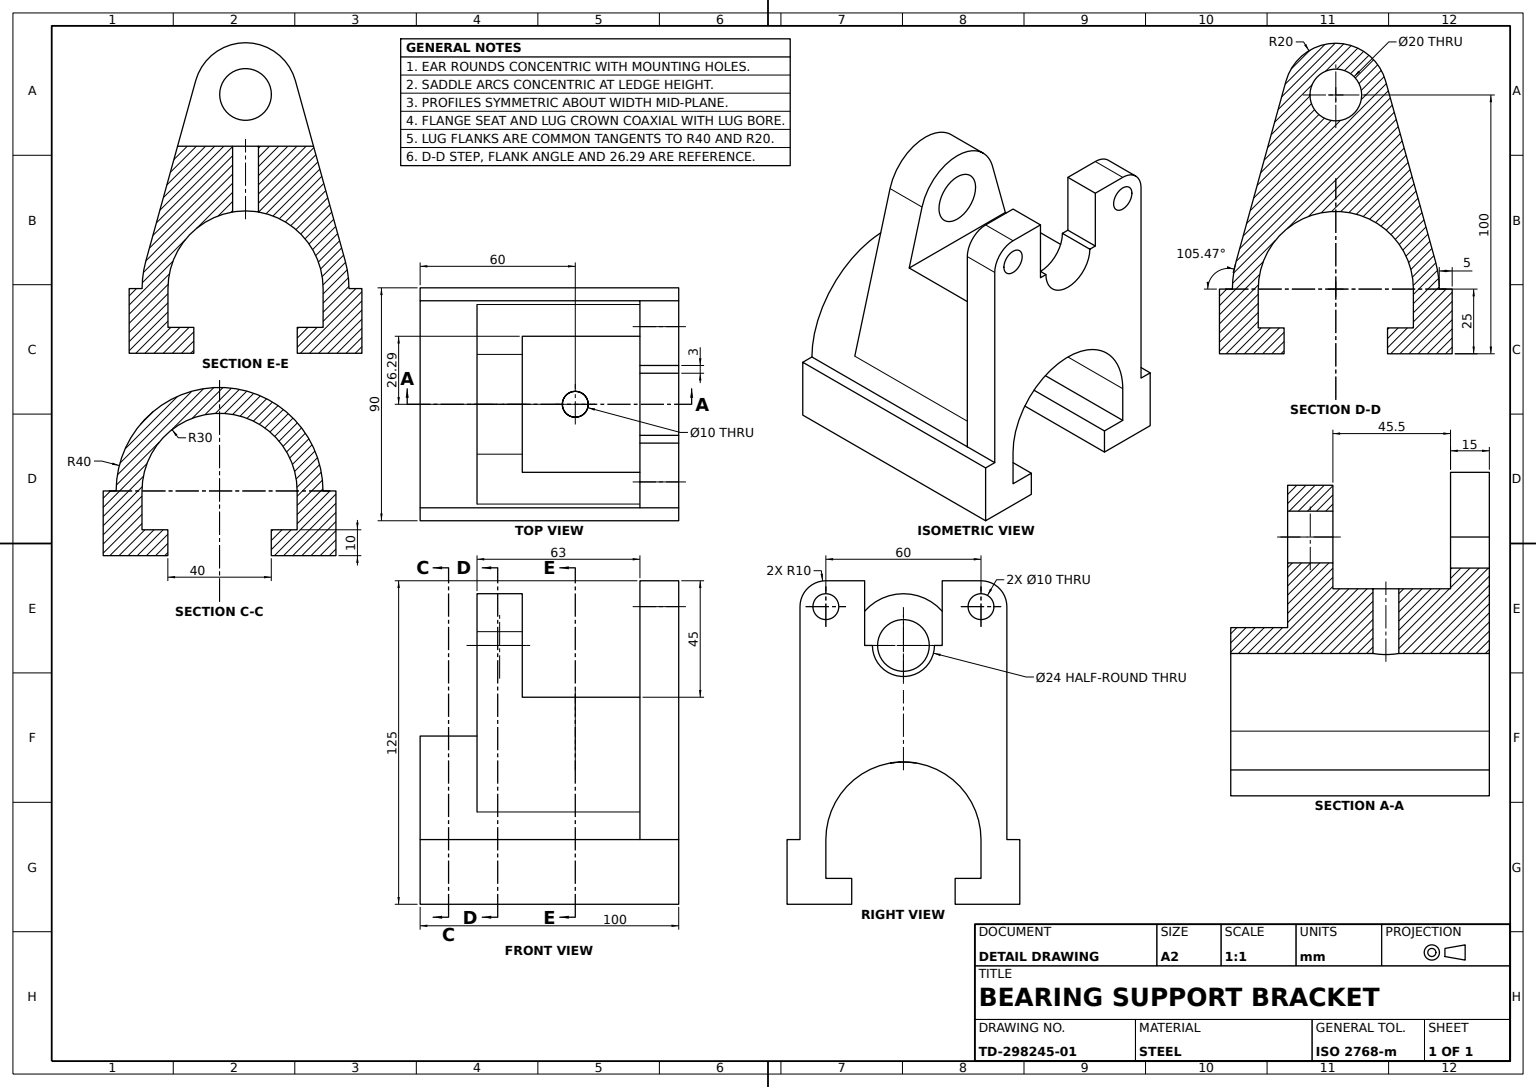
ISO-10303-21;
HEADER;
FILE_DESCRIPTION((''),'2;1');
FILE_NAME('','',(''),(''),'','','');
FILE_SCHEMA(('AUTOMOTIVE_DESIGN'));
ENDSEC;
DATA;
#1=APPLICATION_CONTEXT('');
#2=PRODUCT_CONTEXT('',#1,'mechanical');
#3=PRODUCT('','','',(#2));
#4=PRODUCT_DEFINITION_FORMATION('','',#3);
#5=PRODUCT_DEFINITION_CONTEXT('',#1,'design');
#6=PRODUCT_DEFINITION('','',#4,#5);
#7=PRODUCT_DEFINITION_SHAPE('','',#6);
#8=(LENGTH_UNIT()NAMED_UNIT(*)SI_UNIT(.MILLI.,.METRE.));
#9=(NAMED_UNIT(*)PLANE_ANGLE_UNIT()SI_UNIT($,.RADIAN.));
#10=(NAMED_UNIT(*)SI_UNIT($,.STERADIAN.)SOLID_ANGLE_UNIT());
#11=UNCERTAINTY_MEASURE_WITH_UNIT(LENGTH_MEASURE(1.E-05),#8,'distance_accuracy_value','');
#12=(GEOMETRIC_REPRESENTATION_CONTEXT(3)GLOBAL_UNCERTAINTY_ASSIGNED_CONTEXT((#11))GLOBAL_UNIT_ASSIGNED_CONTEXT((#8,#9,#10))REPRESENTATION_CONTEXT('',''));
#13=CARTESIAN_POINT('',(45.,25.,100.));
#14=VERTEX_POINT('',#13);
#15=CARTESIAN_POINT('',(45.,25.,0.));
#16=VERTEX_POINT('',#15);
#17=DIRECTION('',(0.,0.,-1.));
#18=VECTOR('',#17,1000.);
#19=LINE('',#13,#18);
#20=EDGE_CURVE('',#14,#16,#19,.T.);
#21=ORIENTED_EDGE('',*,*,#20,.T.);
#22=CARTESIAN_POINT('',(40.,25.,0.));
#23=VERTEX_POINT('',#22);
#24=CARTESIAN_POINT('',(0.,25.,0.));
#25=DIRECTION('',(1.,0.,0.));
#26=VECTOR('',#25,1000.);
#27=LINE('',#24,#26);
#28=EDGE_CURVE('',#23,#16,#27,.T.);
#29=ORIENTED_EDGE('',*,*,#28,.F.);
#30=CARTESIAN_POINT('',(40.,25.,15.));
#31=VERTEX_POINT('',#30);
#32=LINE('',#30,#18);
#33=EDGE_CURVE('',#31,#23,#32,.T.);
#34=ORIENTED_EDGE('',*,*,#33,.F.);
#35=CARTESIAN_POINT('',(40.,25.,100.));
#36=VERTEX_POINT('',#35);
#37=LINE('',#35,#18);
#38=EDGE_CURVE('',#36,#31,#37,.T.);
#39=ORIENTED_EDGE('',*,*,#38,.F.);
#40=CARTESIAN_POINT('',(0.,25.,100.));
#41=LINE('',#40,#26);
#42=EDGE_CURVE('',#36,#14,#41,.T.);
#43=ORIENTED_EDGE('',*,*,#42,.T.);
#44=EDGE_LOOP('',(#21,#29,#34,#39,#43));
#45=FACE_OUTER_BOUND('',#44,.T.);
#46=DIRECTION('',(0.,1.,0.));
#47=DIRECTION('',(-1.,0.,0.));
#48=AXIS2_PLACEMENT_3D('',#40,#46,#47);
#49=PLANE('',#48);
#50=ADVANCED_FACE('',(#45),#49,.T.);
#51=CARTESIAN_POINT('',(38.551553,35.666667,15.));
#52=VERTEX_POINT('',#51);
#53=CARTESIAN_POINT('',(0.,25.,15.));
#54=DIRECTION('',(0.,0.,1.));
#55=AXIS2_PLACEMENT_3D('',#53,#54,#25);
#56=CIRCLE('',#55,40.);
#57=EDGE_CURVE('',#31,#52,#56,.T.);
#58=ORIENTED_EDGE('',*,*,#57,.F.);
#59=CARTESIAN_POINT('',(40.,115.,15.));
#60=VERTEX_POINT('',#59);
#61=CARTESIAN_POINT('',(40.,0.,15.));
#62=DIRECTION('',(0.,-1.,0.));
#63=VECTOR('',#62,1000.);
#64=LINE('',#61,#63);
#65=EDGE_CURVE('',#60,#31,#64,.T.);
#66=ORIENTED_EDGE('',*,*,#65,.F.);
#67=CARTESIAN_POINT('',(30.,125.,15.));
#68=VERTEX_POINT('',#67);
#69=CARTESIAN_POINT('',(30.,115.,15.));
#70=AXIS2_PLACEMENT_3D('',#69,#17,#25);
#71=CIRCLE('',#70,10.);
#72=EDGE_CURVE('',#68,#60,#71,.T.);
#73=ORIENTED_EDGE('',*,*,#72,.F.);
#74=CARTESIAN_POINT('',(15.,125.,15.));
#75=VERTEX_POINT('',#74);
#76=CARTESIAN_POINT('',(0.,125.,15.));
#77=LINE('',#76,#26);
#78=EDGE_CURVE('',#75,#68,#77,.T.);
#79=ORIENTED_EDGE('',*,*,#78,.F.);
#80=CARTESIAN_POINT('',(15.,100.,15.));
#81=VERTEX_POINT('',#80);
#82=CARTESIAN_POINT('',(15.,0.,15.));
#83=LINE('',#82,#63);
#84=EDGE_CURVE('',#75,#81,#83,.T.);
#85=ORIENTED_EDGE('',*,*,#84,.T.);
#86=CARTESIAN_POINT('',(12.,100.,15.));
#87=VERTEX_POINT('',#86);
#88=CARTESIAN_POINT('',(0.,100.,15.));
#89=LINE('',#88,#26);
#90=EDGE_CURVE('',#87,#81,#89,.T.);
#91=ORIENTED_EDGE('',*,*,#90,.F.);
#92=CARTESIAN_POINT('',(-12.,100.,15.));
#93=VERTEX_POINT('',#92);
#94=AXIS2_PLACEMENT_3D('',#88,#54,#25);
#95=CIRCLE('',#94,12.);
#96=EDGE_CURVE('',#93,#87,#95,.T.);
#97=ORIENTED_EDGE('',*,*,#96,.F.);
#98=CARTESIAN_POINT('',(-15.,100.,15.));
#99=VERTEX_POINT('',#98);
#100=EDGE_CURVE('',#99,#93,#89,.T.);
#101=ORIENTED_EDGE('',*,*,#100,.F.);
#102=CARTESIAN_POINT('',(-15.,125.,15.));
#103=VERTEX_POINT('',#102);
#104=CARTESIAN_POINT('',(-15.,0.,15.));
#105=LINE('',#104,#63);
#106=EDGE_CURVE('',#103,#99,#105,.T.);
#107=ORIENTED_EDGE('',*,*,#106,.F.);
#108=CARTESIAN_POINT('',(-30.,125.,15.));
#109=VERTEX_POINT('',#108);
#110=EDGE_CURVE('',#109,#103,#77,.T.);
#111=ORIENTED_EDGE('',*,*,#110,.F.);
#112=CARTESIAN_POINT('',(-40.,115.,15.));
#113=VERTEX_POINT('',#112);
#114=CARTESIAN_POINT('',(-30.,115.,15.));
#115=AXIS2_PLACEMENT_3D('',#114,#54,#25);
#116=CIRCLE('',#115,10.);
#117=EDGE_CURVE('',#109,#113,#116,.T.);
#118=ORIENTED_EDGE('',*,*,#117,.T.);
#119=CARTESIAN_POINT('',(-40.,25.,15.));
#120=VERTEX_POINT('',#119);
#121=CARTESIAN_POINT('',(-40.,0.,15.));
#122=LINE('',#121,#63);
#123=EDGE_CURVE('',#113,#120,#122,.T.);
#124=ORIENTED_EDGE('',*,*,#123,.T.);
#125=CARTESIAN_POINT('',(-38.551553,35.666667,15.));
#126=VERTEX_POINT('',#125);
#127=EDGE_CURVE('',#126,#120,#56,.T.);
#128=ORIENTED_EDGE('',*,*,#127,.F.);
#129=CARTESIAN_POINT('',(-26.28515,80.,15.));
#130=VERTEX_POINT('',#129);
#131=CARTESIAN_POINT('',(-19.275776,105.333333,15.));
#132=DIRECTION('',(-0.266666667,-0.96378882,0.));
#133=VECTOR('',#132,1000.);
#134=LINE('',#131,#133);
#135=EDGE_CURVE('',#130,#126,#134,.T.);
#136=ORIENTED_EDGE('',*,*,#135,.F.);
#137=CARTESIAN_POINT('',(26.28515,80.,15.));
#138=VERTEX_POINT('',#137);
#139=CARTESIAN_POINT('',(-45.,80.,15.));
#140=LINE('',#139,#26);
#141=EDGE_CURVE('',#130,#138,#140,.T.);
#142=ORIENTED_EDGE('',*,*,#141,.T.);
#143=CARTESIAN_POINT('',(19.275776,105.333333,15.));
#144=DIRECTION('',(-0.266666667,0.96378882,0.));
#145=VECTOR('',#144,1000.);
#146=LINE('',#143,#145);
#147=EDGE_CURVE('',#52,#138,#146,.T.);
#148=ORIENTED_EDGE('',*,*,#147,.F.);
#149=EDGE_LOOP('',(#58,#66,#73,#79,#85,#91,#97,#101,#107,#111,#118,#124,#128,#136,#142,#148));
#150=FACE_OUTER_BOUND('',#149,.T.);
#151=CARTESIAN_POINT('',(-35.,115.,15.));
#152=VERTEX_POINT('',#151);
#153=CARTESIAN_POINT('',(-25.,115.,15.));
#154=VERTEX_POINT('',#153);
#155=CIRCLE('',#115,5.);
#156=EDGE_CURVE('',#152,#154,#155,.T.);
#157=ORIENTED_EDGE('',*,*,#156,.F.);
#158=EDGE_CURVE('',#154,#152,#155,.T.);
#159=ORIENTED_EDGE('',*,*,#158,.F.);
#160=EDGE_LOOP('',(#157,#159));
#161=FACE_BOUND('',#160,.T.);
#162=CARTESIAN_POINT('',(25.,115.,15.));
#163=VERTEX_POINT('',#162);
#164=CARTESIAN_POINT('',(35.,115.,15.));
#165=VERTEX_POINT('',#164);
#166=CIRCLE('',#70,5.);
#167=EDGE_CURVE('',#163,#165,#166,.T.);
#168=ORIENTED_EDGE('',*,*,#167,.T.);
#169=EDGE_CURVE('',#165,#163,#166,.T.);
#170=ORIENTED_EDGE('',*,*,#169,.T.);
#171=EDGE_LOOP('',(#168,#170));
#172=FACE_BOUND('',#171,.T.);
#173=CARTESIAN_POINT('',(0.,0.,15.));
#174=AXIS2_PLACEMENT_3D('',#173,#54,#25);
#175=PLANE('',#174);
#176=ADVANCED_FACE('',(#150,#161,#172),#175,.T.);
#177=CARTESIAN_POINT('',(40.,115.,0.));
#178=VERTEX_POINT('',#177);
#179=LINE('',#59,#18);
#180=EDGE_CURVE('',#60,#178,#179,.T.);
#181=ORIENTED_EDGE('',*,*,#180,.F.);
#182=ORIENTED_EDGE('',*,*,#65,.T.);
#183=ORIENTED_EDGE('',*,*,#33,.T.);
#184=CARTESIAN_POINT('',(40.,0.,0.));
#185=LINE('',#184,#63);
#186=EDGE_CURVE('',#178,#23,#185,.T.);
#187=ORIENTED_EDGE('',*,*,#186,.F.);
#188=EDGE_LOOP('',(#181,#182,#183,#187));
#189=FACE_OUTER_BOUND('',#188,.T.);
#190=AXIS2_PLACEMENT_3D('',#61,#25,#46);
#191=PLANE('',#190);
#192=ADVANCED_FACE('',(#189),#191,.T.);
#193=CARTESIAN_POINT('',(20.,0.,0.));
#194=VERTEX_POINT('',#193);
#195=CARTESIAN_POINT('',(20.,10.,0.));
#196=VERTEX_POINT('',#195);
#197=VECTOR('',#46,1000.);
#198=LINE('',#193,#197);
#199=EDGE_CURVE('',#194,#196,#198,.T.);
#200=ORIENTED_EDGE('',*,*,#199,.F.);
#201=CARTESIAN_POINT('',(20.,0.,100.));
#202=VERTEX_POINT('',#201);
#203=LINE('',#201,#18);
#204=EDGE_CURVE('',#202,#194,#203,.T.);
#205=ORIENTED_EDGE('',*,*,#204,.F.);
#206=CARTESIAN_POINT('',(20.,10.,100.));
#207=VERTEX_POINT('',#206);
#208=LINE('',#201,#197);
#209=EDGE_CURVE('',#202,#207,#208,.T.);
#210=ORIENTED_EDGE('',*,*,#209,.T.);
#211=LINE('',#206,#18);
#212=EDGE_CURVE('',#207,#196,#211,.T.);
#213=ORIENTED_EDGE('',*,*,#212,.T.);
#214=EDGE_LOOP('',(#200,#205,#210,#213));
#215=FACE_OUTER_BOUND('',#214,.T.);
#216=AXIS2_PLACEMENT_3D('',#201,#47,#62);
#217=PLANE('',#216);
#218=ADVANCED_FACE('',(#215),#217,.T.);
#219=CARTESIAN_POINT('',(30.,25.,100.));
#220=VERTEX_POINT('',#219);
#221=CARTESIAN_POINT('',(30.,25.,0.));
#222=VERTEX_POINT('',#221);
#223=LINE('',#219,#18);
#224=EDGE_CURVE('',#220,#222,#223,.T.);
#225=ORIENTED_EDGE('',*,*,#224,.T.);
#226=CARTESIAN_POINT('',(30.,10.,0.));
#227=VERTEX_POINT('',#226);
#228=CARTESIAN_POINT('',(30.,0.,0.));
#229=LINE('',#228,#197);
#230=EDGE_CURVE('',#227,#222,#229,.T.);
#231=ORIENTED_EDGE('',*,*,#230,.F.);
#232=CARTESIAN_POINT('',(30.,10.,100.));
#233=VERTEX_POINT('',#232);
#234=LINE('',#232,#18);
#235=EDGE_CURVE('',#233,#227,#234,.T.);
#236=ORIENTED_EDGE('',*,*,#235,.F.);
#237=CARTESIAN_POINT('',(30.,0.,100.));
#238=LINE('',#237,#197);
#239=EDGE_CURVE('',#233,#220,#238,.T.);
#240=ORIENTED_EDGE('',*,*,#239,.T.);
#241=EDGE_LOOP('',(#225,#231,#236,#240));
#242=FACE_OUTER_BOUND('',#241,.T.);
#243=AXIS2_PLACEMENT_3D('',#237,#47,#54);
#244=PLANE('',#243);
#245=ADVANCED_FACE('',(#242),#244,.T.);
#246=CARTESIAN_POINT('',(35.,115.,0.));
#247=VERTEX_POINT('',#246);
#248=CARTESIAN_POINT('',(25.,115.,0.));
#249=VERTEX_POINT('',#248);
#250=CARTESIAN_POINT('',(30.,115.,0.));
#251=AXIS2_PLACEMENT_3D('',#250,#17,#25);
#252=CIRCLE('',#251,5.);
#253=EDGE_CURVE('',#247,#249,#252,.T.);
#254=ORIENTED_EDGE('',*,*,#253,.T.);
#255=LINE('',#162,#18);
#256=EDGE_CURVE('',#163,#249,#255,.T.);
#257=ORIENTED_EDGE('',*,*,#256,.F.);
#258=ORIENTED_EDGE('',*,*,#169,.F.);
#259=LINE('',#164,#18);
#260=EDGE_CURVE('',#165,#247,#259,.T.);
#261=ORIENTED_EDGE('',*,*,#260,.T.);
#262=EDGE_LOOP('',(#254,#257,#258,#261));
#263=FACE_OUTER_BOUND('',#262,.T.);
#264=AXIS2_PLACEMENT_3D('',#69,#17,#47);
#265=CYLINDRICAL_SURFACE('',#264,5.);
#266=ADVANCED_FACE('',(#263),#265,.F.);
#267=CARTESIAN_POINT('',(-10.,100.,78.));
#268=VERTEX_POINT('',#267);
#269=CARTESIAN_POINT('',(10.,100.,78.));
#270=VERTEX_POINT('',#269);
#271=CARTESIAN_POINT('',(0.,100.,78.));
#272=AXIS2_PLACEMENT_3D('',#271,#54,#25);
#273=CIRCLE('',#272,10.);
#274=EDGE_CURVE('',#268,#270,#273,.T.);
#275=ORIENTED_EDGE('',*,*,#274,.F.);
#276=EDGE_CURVE('',#270,#268,#273,.T.);
#277=ORIENTED_EDGE('',*,*,#276,.F.);
#278=EDGE_LOOP('',(#275,#277));
#279=FACE_BOUND('',#278,.T.);
#280=CARTESIAN_POINT('',(38.551553,35.666667,78.));
#281=VERTEX_POINT('',#280);
#282=CARTESIAN_POINT('',(19.275776,105.333333,78.));
#283=VERTEX_POINT('',#282);
#284=LINE('',#282,#145);
#285=EDGE_CURVE('',#281,#283,#284,.T.);
#286=ORIENTED_EDGE('',*,*,#285,.T.);
#287=CARTESIAN_POINT('',(-19.275776,105.333333,78.));
#288=VERTEX_POINT('',#287);
#289=CIRCLE('',#272,20.);
#290=EDGE_CURVE('',#283,#288,#289,.T.);
#291=ORIENTED_EDGE('',*,*,#290,.T.);
#292=CARTESIAN_POINT('',(-38.551553,35.666667,78.));
#293=VERTEX_POINT('',#292);
#294=LINE('',#287,#133);
#295=EDGE_CURVE('',#288,#293,#294,.T.);
#296=ORIENTED_EDGE('',*,*,#295,.T.);
#297=CARTESIAN_POINT('',(0.,25.,78.));
#298=AXIS2_PLACEMENT_3D('',#297,#17,#25);
#299=CIRCLE('',#298,40.);
#300=EDGE_CURVE('',#293,#281,#299,.T.);
#301=ORIENTED_EDGE('',*,*,#300,.T.);
#302=EDGE_LOOP('',(#286,#291,#296,#301));
#303=FACE_OUTER_BOUND('',#302,.T.);
#304=AXIS2_PLACEMENT_3D('',#297,#54,#25);
#305=PLANE('',#304);
#306=ADVANCED_FACE('',(#279,#303),#305,.T.);
#307=CARTESIAN_POINT('',(45.,0.,100.));
#308=VERTEX_POINT('',#307);
#309=CARTESIAN_POINT('',(45.,0.,0.));
#310=VERTEX_POINT('',#309);
#311=LINE('',#307,#18);
#312=EDGE_CURVE('',#308,#310,#311,.T.);
#313=ORIENTED_EDGE('',*,*,#312,.T.);
#314=LINE('',#309,#63);
#315=EDGE_CURVE('',#16,#310,#314,.T.);
#316=ORIENTED_EDGE('',*,*,#315,.F.);
#317=ORIENTED_EDGE('',*,*,#20,.F.);
#318=LINE('',#307,#63);
#319=EDGE_CURVE('',#14,#308,#318,.T.);
#320=ORIENTED_EDGE('',*,*,#319,.T.);
#321=EDGE_LOOP('',(#313,#316,#317,#320));
#322=FACE_OUTER_BOUND('',#321,.T.);
#323=AXIS2_PLACEMENT_3D('',#307,#25,#17);
#324=PLANE('',#323);
#325=ADVANCED_FACE('',(#322),#324,.T.);
#326=ORIENTED_EDGE('',*,*,#312,.F.);
#327=CARTESIAN_POINT('',(0.,0.,100.));
#328=LINE('',#327,#26);
#329=EDGE_CURVE('',#202,#308,#328,.T.);
#330=ORIENTED_EDGE('',*,*,#329,.F.);
#331=ORIENTED_EDGE('',*,*,#204,.T.);
#332=CARTESIAN_POINT('',(0.,0.,0.));
#333=LINE('',#332,#26);
#334=EDGE_CURVE('',#194,#310,#333,.T.);
#335=ORIENTED_EDGE('',*,*,#334,.T.);
#336=EDGE_LOOP('',(#326,#330,#331,#335));
#337=FACE_OUTER_BOUND('',#336,.T.);
#338=AXIS2_PLACEMENT_3D('',#327,#46,#47);
#339=PLANE('',#338);
#340=ADVANCED_FACE('',(#337),#339,.F.);
#341=CARTESIAN_POINT('',(-10.,100.,60.5));
#342=VERTEX_POINT('',#341);
#343=LINE('',#267,#18);
#344=EDGE_CURVE('',#268,#342,#343,.T.);
#345=ORIENTED_EDGE('',*,*,#344,.T.);
#346=CARTESIAN_POINT('',(10.,100.,60.5));
#347=VERTEX_POINT('',#346);
#348=CARTESIAN_POINT('',(0.,100.,60.5));
#349=AXIS2_PLACEMENT_3D('',#348,#54,#62);
#350=CIRCLE('',#349,10.);
#351=EDGE_CURVE('',#347,#342,#350,.T.);
#352=ORIENTED_EDGE('',*,*,#351,.F.);
#353=LINE('',#269,#18);
#354=EDGE_CURVE('',#270,#347,#353,.T.);
#355=ORIENTED_EDGE('',*,*,#354,.F.);
#356=ORIENTED_EDGE('',*,*,#276,.T.);
#357=EDGE_LOOP('',(#345,#352,#355,#356));
#358=FACE_OUTER_BOUND('',#357,.T.);
#359=AXIS2_PLACEMENT_3D('',#271,#17,#47);
#360=CYLINDRICAL_SURFACE('',#359,10.);
#361=ADVANCED_FACE('',(#358),#360,.F.);
#362=CARTESIAN_POINT('',(-45.,25.,100.));
#363=VERTEX_POINT('',#362);
#364=CARTESIAN_POINT('',(-45.,0.,100.));
#365=VERTEX_POINT('',#364);
#366=LINE('',#364,#63);
#367=EDGE_CURVE('',#363,#365,#366,.T.);
#368=ORIENTED_EDGE('',*,*,#367,.F.);
#369=CARTESIAN_POINT('',(-45.,25.,0.));
#370=VERTEX_POINT('',#369);
#371=LINE('',#362,#18);
#372=EDGE_CURVE('',#363,#370,#371,.T.);
#373=ORIENTED_EDGE('',*,*,#372,.T.);
#374=CARTESIAN_POINT('',(-45.,0.,0.));
#375=VERTEX_POINT('',#374);
#376=LINE('',#374,#63);
#377=EDGE_CURVE('',#370,#375,#376,.T.);
#378=ORIENTED_EDGE('',*,*,#377,.T.);
#379=LINE('',#364,#18);
#380=EDGE_CURVE('',#365,#375,#379,.T.);
#381=ORIENTED_EDGE('',*,*,#380,.F.);
#382=EDGE_LOOP('',(#368,#373,#378,#381));
#383=FACE_OUTER_BOUND('',#382,.T.);
#384=AXIS2_PLACEMENT_3D('',#364,#25,#17);
#385=PLANE('',#384);
#386=ADVANCED_FACE('',(#383),#385,.F.);
#387=CARTESIAN_POINT('',(-19.275776,105.333333,60.5));
#388=VERTEX_POINT('',#387);
#389=LINE('',#287,#18);
#390=EDGE_CURVE('',#288,#388,#389,.T.);
#391=ORIENTED_EDGE('',*,*,#390,.T.);
#392=CARTESIAN_POINT('',(-26.28515,80.,60.5));
#393=VERTEX_POINT('',#392);
#394=LINE('',#387,#133);
#395=EDGE_CURVE('',#388,#393,#394,.T.);
#396=ORIENTED_EDGE('',*,*,#395,.T.);
#397=CARTESIAN_POINT('',(-26.28515,80.,78.));
#398=LINE('',#397,#18);
#399=EDGE_CURVE('',#393,#130,#398,.T.);
#400=ORIENTED_EDGE('',*,*,#399,.T.);
#401=ORIENTED_EDGE('',*,*,#135,.T.);
#402=LINE('',#292,#18);
#403=EDGE_CURVE('',#293,#126,#402,.T.);
#404=ORIENTED_EDGE('',*,*,#403,.F.);
#405=ORIENTED_EDGE('',*,*,#295,.F.);
#406=EDGE_LOOP('',(#391,#396,#400,#401,#404,#405));
#407=FACE_OUTER_BOUND('',#406,.T.);
#408=DIRECTION('',(0.96378882,-0.266666667,0.));
#409=DIRECTION('',(0.266666667,0.96378882,0.));
#410=AXIS2_PLACEMENT_3D('',#287,#408,#409);
#411=PLANE('',#410);
#412=ADVANCED_FACE('',(#407),#411,.F.);
#413=CARTESIAN_POINT('',(0.,10.,100.));
#414=LINE('',#413,#26);
#415=EDGE_CURVE('',#207,#233,#414,.T.);
#416=ORIENTED_EDGE('',*,*,#415,.F.);
#417=ORIENTED_EDGE('',*,*,#209,.F.);
#418=ORIENTED_EDGE('',*,*,#329,.T.);
#419=ORIENTED_EDGE('',*,*,#319,.F.);
#420=ORIENTED_EDGE('',*,*,#42,.F.);
#421=CARTESIAN_POINT('',(-40.,25.,100.));
#422=VERTEX_POINT('',#421);
#423=AXIS2_PLACEMENT_3D('',#40,#54,#25);
#424=CIRCLE('',#423,40.);
#425=EDGE_CURVE('',#36,#422,#424,.T.);
#426=ORIENTED_EDGE('',*,*,#425,.T.);
#427=VECTOR('',#47,1000.);
#428=LINE('',#40,#427);
#429=EDGE_CURVE('',#422,#363,#428,.T.);
#430=ORIENTED_EDGE('',*,*,#429,.T.);
#431=ORIENTED_EDGE('',*,*,#367,.T.);
#432=CARTESIAN_POINT('',(-20.,0.,100.));
#433=VERTEX_POINT('',#432);
#434=EDGE_CURVE('',#365,#433,#328,.T.);
#435=ORIENTED_EDGE('',*,*,#434,.T.);
#436=CARTESIAN_POINT('',(-20.,10.,100.));
#437=VERTEX_POINT('',#436);
#438=LINE('',#432,#197);
#439=EDGE_CURVE('',#433,#437,#438,.T.);
#440=ORIENTED_EDGE('',*,*,#439,.T.);
#441=CARTESIAN_POINT('',(-30.,10.,100.));
#442=VERTEX_POINT('',#441);
#443=LINE('',#413,#427);
#444=EDGE_CURVE('',#437,#442,#443,.T.);
#445=ORIENTED_EDGE('',*,*,#444,.T.);
#446=CARTESIAN_POINT('',(-30.,25.,100.));
#447=VERTEX_POINT('',#446);
#448=CARTESIAN_POINT('',(-30.,0.,100.));
#449=LINE('',#448,#197);
#450=EDGE_CURVE('',#442,#447,#449,.T.);
#451=ORIENTED_EDGE('',*,*,#450,.T.);
#452=CIRCLE('',#423,30.);
#453=EDGE_CURVE('',#220,#447,#452,.T.);
#454=ORIENTED_EDGE('',*,*,#453,.F.);
#455=ORIENTED_EDGE('',*,*,#239,.F.);
#456=EDGE_LOOP('',(#416,#417,#418,#419,#420,#426,#430,#431,#435,#440,#445,#451,#454,#455));
#457=FACE_OUTER_BOUND('',#456,.T.);
#458=AXIS2_PLACEMENT_3D('',#327,#54,#25);
#459=PLANE('',#458);
#460=ADVANCED_FACE('',(#457),#459,.T.);
#461=ORIENTED_EDGE('',*,*,#351,.T.);
#462=EDGE_CURVE('',#342,#347,#350,.T.);
#463=ORIENTED_EDGE('',*,*,#462,.T.);
#464=EDGE_LOOP('',(#461,#463));
#465=FACE_BOUND('',#464,.T.);
#466=CARTESIAN_POINT('',(26.28515,80.,60.5));
#467=VERTEX_POINT('',#466);
#468=CARTESIAN_POINT('',(19.275776,105.333333,60.5));
#469=VERTEX_POINT('',#468);
#470=LINE('',#468,#145);
#471=EDGE_CURVE('',#467,#469,#470,.T.);
#472=ORIENTED_EDGE('',*,*,#471,.F.);
#473=CARTESIAN_POINT('',(-45.,80.,60.5));
#474=LINE('',#473,#26);
#475=EDGE_CURVE('',#393,#467,#474,.T.);
#476=ORIENTED_EDGE('',*,*,#475,.F.);
#477=ORIENTED_EDGE('',*,*,#395,.F.);
#478=CIRCLE('',#349,20.);
#479=EDGE_CURVE('',#469,#388,#478,.T.);
#480=ORIENTED_EDGE('',*,*,#479,.F.);
#481=EDGE_LOOP('',(#472,#476,#477,#480));
#482=FACE_OUTER_BOUND('',#481,.T.);
#483=CARTESIAN_POINT('',(-45.,125.,60.5));
#484=AXIS2_PLACEMENT_3D('',#483,#54,#62);
#485=PLANE('',#484);
#486=ADVANCED_FACE('',(#465,#482),#485,.F.);
#487=CARTESIAN_POINT('',(-30.,125.,0.));
#488=VERTEX_POINT('',#487);
#489=CARTESIAN_POINT('',(-15.,125.,0.));
#490=VERTEX_POINT('',#489);
#491=CARTESIAN_POINT('',(0.,125.,0.));
#492=LINE('',#491,#26);
#493=EDGE_CURVE('',#488,#490,#492,.T.);
#494=ORIENTED_EDGE('',*,*,#493,.F.);
#495=LINE('',#108,#18);
#496=EDGE_CURVE('',#109,#488,#495,.T.);
#497=ORIENTED_EDGE('',*,*,#496,.F.);
#498=ORIENTED_EDGE('',*,*,#110,.T.);
#499=LINE('',#102,#18);
#500=EDGE_CURVE('',#103,#490,#499,.T.);
#501=ORIENTED_EDGE('',*,*,#500,.T.);
#502=EDGE_LOOP('',(#494,#497,#498,#501));
#503=FACE_OUTER_BOUND('',#502,.T.);
#504=AXIS2_PLACEMENT_3D('',#76,#46,#47);
#505=PLANE('',#504);
#506=ADVANCED_FACE('',(#503),#505,.T.);
#507=CARTESIAN_POINT('',(-40.,115.,0.));
#508=VERTEX_POINT('',#507);
#509=LINE('',#112,#18);
#510=EDGE_CURVE('',#113,#508,#509,.T.);
#511=ORIENTED_EDGE('',*,*,#510,.T.);
#512=CARTESIAN_POINT('',(-40.,25.,0.));
#513=VERTEX_POINT('',#512);
#514=CARTESIAN_POINT('',(-40.,0.,0.));
#515=LINE('',#514,#63);
#516=EDGE_CURVE('',#508,#513,#515,.T.);
#517=ORIENTED_EDGE('',*,*,#516,.T.);
#518=LINE('',#119,#18);
#519=EDGE_CURVE('',#120,#513,#518,.T.);
#520=ORIENTED_EDGE('',*,*,#519,.F.);
#521=ORIENTED_EDGE('',*,*,#123,.F.);
#522=EDGE_LOOP('',(#511,#517,#520,#521));
#523=FACE_OUTER_BOUND('',#522,.T.);
#524=AXIS2_PLACEMENT_3D('',#121,#25,#17);
#525=PLANE('',#524);
#526=ADVANCED_FACE('',(#523),#525,.F.);
#527=CARTESIAN_POINT('',(12.,100.,0.));
#528=VERTEX_POINT('',#527);
#529=CARTESIAN_POINT('',(15.,100.,0.));
#530=VERTEX_POINT('',#529);
#531=CARTESIAN_POINT('',(0.,100.,0.));
#532=LINE('',#531,#26);
#533=EDGE_CURVE('',#528,#530,#532,.T.);
#534=ORIENTED_EDGE('',*,*,#533,.F.);
#535=LINE('',#86,#18);
#536=EDGE_CURVE('',#87,#528,#535,.T.);
#537=ORIENTED_EDGE('',*,*,#536,.F.);
#538=ORIENTED_EDGE('',*,*,#90,.T.);
#539=LINE('',#80,#18);
#540=EDGE_CURVE('',#81,#530,#539,.T.);
#541=ORIENTED_EDGE('',*,*,#540,.T.);
#542=EDGE_LOOP('',(#534,#537,#538,#541));
#543=FACE_OUTER_BOUND('',#542,.T.);
#544=AXIS2_PLACEMENT_3D('',#88,#46,#54);
#545=PLANE('',#544);
#546=ADVANCED_FACE('',(#543),#545,.T.);
#547=EDGE_CURVE('',#249,#247,#252,.T.);
#548=ORIENTED_EDGE('',*,*,#547,.T.);
#549=ORIENTED_EDGE('',*,*,#260,.F.);
#550=ORIENTED_EDGE('',*,*,#167,.F.);
#551=ORIENTED_EDGE('',*,*,#256,.T.);
#552=EDGE_LOOP('',(#548,#549,#550,#551));
#553=FACE_OUTER_BOUND('',#552,.T.);
#554=ADVANCED_FACE('',(#553),#265,.F.);
#555=CARTESIAN_POINT('',(-20.,0.,0.));
#556=VERTEX_POINT('',#555);
#557=CARTESIAN_POINT('',(-20.,10.,0.));
#558=VERTEX_POINT('',#557);
#559=LINE('',#555,#197);
#560=EDGE_CURVE('',#556,#558,#559,.T.);
#561=ORIENTED_EDGE('',*,*,#560,.T.);
#562=LINE('',#436,#18);
#563=EDGE_CURVE('',#437,#558,#562,.T.);
#564=ORIENTED_EDGE('',*,*,#563,.F.);
#565=ORIENTED_EDGE('',*,*,#439,.F.);
#566=LINE('',#432,#18);
#567=EDGE_CURVE('',#433,#556,#566,.T.);
#568=ORIENTED_EDGE('',*,*,#567,.T.);
#569=EDGE_LOOP('',(#561,#564,#565,#568));
#570=FACE_OUTER_BOUND('',#569,.T.);
#571=AXIS2_PLACEMENT_3D('',#432,#47,#54);
#572=PLANE('',#571);
#573=ADVANCED_FACE('',(#570),#572,.F.);
#574=ORIENTED_EDGE('',*,*,#38,.T.);
#575=ORIENTED_EDGE('',*,*,#57,.T.);
#576=LINE('',#280,#18);
#577=EDGE_CURVE('',#281,#52,#576,.T.);
#578=ORIENTED_EDGE('',*,*,#577,.F.);
#579=ORIENTED_EDGE('',*,*,#300,.F.);
#580=ORIENTED_EDGE('',*,*,#403,.T.);
#581=ORIENTED_EDGE('',*,*,#127,.T.);
#582=LINE('',#421,#18);
#583=EDGE_CURVE('',#422,#120,#582,.T.);
#584=ORIENTED_EDGE('',*,*,#583,.F.);
#585=ORIENTED_EDGE('',*,*,#425,.F.);
#586=EDGE_LOOP('',(#574,#575,#578,#579,#580,#581,#584,#585));
#587=FACE_OUTER_BOUND('',#586,.T.);
#588=AXIS2_PLACEMENT_3D('',#40,#17,#47);
#589=CYLINDRICAL_SURFACE('',#588,40.);
#590=ADVANCED_FACE('',(#587),#589,.T.);
#591=ORIENTED_EDGE('',*,*,#235,.T.);
#592=CARTESIAN_POINT('',(0.,10.,0.));
#593=LINE('',#592,#26);
#594=EDGE_CURVE('',#196,#227,#593,.T.);
#595=ORIENTED_EDGE('',*,*,#594,.F.);
#596=ORIENTED_EDGE('',*,*,#212,.F.);
#597=ORIENTED_EDGE('',*,*,#415,.T.);
#598=EDGE_LOOP('',(#591,#595,#596,#597));
#599=FACE_OUTER_BOUND('',#598,.T.);
#600=AXIS2_PLACEMENT_3D('',#413,#46,#54);
#601=PLANE('',#600);
#602=ADVANCED_FACE('',(#599),#601,.T.);
#603=ORIENTED_EDGE('',*,*,#540,.F.);
#604=ORIENTED_EDGE('',*,*,#84,.F.);
#605=CARTESIAN_POINT('',(15.,125.,0.));
#606=VERTEX_POINT('',#605);
#607=LINE('',#74,#18);
#608=EDGE_CURVE('',#75,#606,#607,.T.);
#609=ORIENTED_EDGE('',*,*,#608,.T.);
#610=CARTESIAN_POINT('',(15.,0.,0.));
#611=LINE('',#610,#63);
#612=EDGE_CURVE('',#606,#530,#611,.T.);
#613=ORIENTED_EDGE('',*,*,#612,.T.);
#614=EDGE_LOOP('',(#603,#604,#609,#613));
#615=FACE_OUTER_BOUND('',#614,.T.);
#616=AXIS2_PLACEMENT_3D('',#82,#25,#46);
#617=PLANE('',#616);
#618=ADVANCED_FACE('',(#615),#617,.F.);
#619=ORIENTED_EDGE('',*,*,#547,.F.);
#620=ORIENTED_EDGE('',*,*,#253,.F.);
#621=EDGE_LOOP('',(#619,#620));
#622=FACE_BOUND('',#621,.T.);
#623=CARTESIAN_POINT('',(-35.,115.,0.));
#624=VERTEX_POINT('',#623);
#625=CARTESIAN_POINT('',(-25.,115.,0.));
#626=VERTEX_POINT('',#625);
#627=CARTESIAN_POINT('',(-30.,115.,0.));
#628=AXIS2_PLACEMENT_3D('',#627,#54,#25);
#629=CIRCLE('',#628,5.);
#630=EDGE_CURVE('',#624,#626,#629,.T.);
#631=ORIENTED_EDGE('',*,*,#630,.T.);
#632=EDGE_CURVE('',#626,#624,#629,.T.);
#633=ORIENTED_EDGE('',*,*,#632,.T.);
#634=EDGE_LOOP('',(#631,#633));
#635=FACE_BOUND('',#634,.T.);
#636=CARTESIAN_POINT('',(30.,125.,0.));
#637=VERTEX_POINT('',#636);
#638=CIRCLE('',#251,10.);
#639=EDGE_CURVE('',#637,#178,#638,.T.);
#640=ORIENTED_EDGE('',*,*,#639,.T.);
#641=ORIENTED_EDGE('',*,*,#186,.T.);
#642=ORIENTED_EDGE('',*,*,#28,.T.);
#643=ORIENTED_EDGE('',*,*,#315,.T.);
#644=ORIENTED_EDGE('',*,*,#334,.F.);
#645=ORIENTED_EDGE('',*,*,#199,.T.);
#646=ORIENTED_EDGE('',*,*,#594,.T.);
#647=ORIENTED_EDGE('',*,*,#230,.T.);
#648=CARTESIAN_POINT('',(-30.,25.,0.));
#649=VERTEX_POINT('',#648);
#650=AXIS2_PLACEMENT_3D('',#24,#54,#25);
#651=CIRCLE('',#650,30.);
#652=EDGE_CURVE('',#222,#649,#651,.T.);
#653=ORIENTED_EDGE('',*,*,#652,.T.);
#654=CARTESIAN_POINT('',(-30.,10.,0.));
#655=VERTEX_POINT('',#654);
#656=CARTESIAN_POINT('',(-30.,0.,0.));
#657=LINE('',#656,#197);
#658=EDGE_CURVE('',#655,#649,#657,.T.);
#659=ORIENTED_EDGE('',*,*,#658,.F.);
#660=LINE('',#592,#427);
#661=EDGE_CURVE('',#558,#655,#660,.T.);
#662=ORIENTED_EDGE('',*,*,#661,.F.);
#663=ORIENTED_EDGE('',*,*,#560,.F.);
#664=EDGE_CURVE('',#375,#556,#333,.T.);
#665=ORIENTED_EDGE('',*,*,#664,.F.);
#666=ORIENTED_EDGE('',*,*,#377,.F.);
#667=LINE('',#24,#427);
#668=EDGE_CURVE('',#513,#370,#667,.T.);
#669=ORIENTED_EDGE('',*,*,#668,.F.);
#670=ORIENTED_EDGE('',*,*,#516,.F.);
#671=CIRCLE('',#628,10.);
#672=EDGE_CURVE('',#488,#508,#671,.T.);
#673=ORIENTED_EDGE('',*,*,#672,.F.);
#674=ORIENTED_EDGE('',*,*,#493,.T.);
#675=CARTESIAN_POINT('',(-15.,100.,0.));
#676=VERTEX_POINT('',#675);
#677=CARTESIAN_POINT('',(-15.,0.,0.));
#678=LINE('',#677,#63);
#679=EDGE_CURVE('',#490,#676,#678,.T.);
#680=ORIENTED_EDGE('',*,*,#679,.T.);
#681=CARTESIAN_POINT('',(-12.,100.,0.));
#682=VERTEX_POINT('',#681);
#683=EDGE_CURVE('',#676,#682,#532,.T.);
#684=ORIENTED_EDGE('',*,*,#683,.T.);
#685=AXIS2_PLACEMENT_3D('',#531,#54,#25);
#686=CIRCLE('',#685,12.);
#687=EDGE_CURVE('',#682,#528,#686,.T.);
#688=ORIENTED_EDGE('',*,*,#687,.T.);
#689=ORIENTED_EDGE('',*,*,#533,.T.);
#690=ORIENTED_EDGE('',*,*,#612,.F.);
#691=EDGE_CURVE('',#606,#637,#492,.T.);
#692=ORIENTED_EDGE('',*,*,#691,.T.);
#693=EDGE_LOOP('',(#640,#641,#642,#643,#644,#645,#646,#647,#653,#659,#662,#663,#665,#666,#669,#670,#673,#674,#680,#684,#688,#689,#690,#692));
#694=FACE_OUTER_BOUND('',#693,.T.);
#695=AXIS2_PLACEMENT_3D('',#332,#54,#25);
#696=PLANE('',#695);
#697=ADVANCED_FACE('',(#622,#635,#694),#696,.F.);
#698=ORIENTED_EDGE('',*,*,#658,.T.);
#699=LINE('',#446,#18);
#700=EDGE_CURVE('',#447,#649,#699,.T.);
#701=ORIENTED_EDGE('',*,*,#700,.F.);
#702=ORIENTED_EDGE('',*,*,#450,.F.);
#703=LINE('',#441,#18);
#704=EDGE_CURVE('',#442,#655,#703,.T.);
#705=ORIENTED_EDGE('',*,*,#704,.T.);
#706=EDGE_LOOP('',(#698,#701,#702,#705));
#707=FACE_OUTER_BOUND('',#706,.T.);
#708=AXIS2_PLACEMENT_3D('',#448,#47,#54);
#709=PLANE('',#708);
#710=ADVANCED_FACE('',(#707),#709,.F.);
#711=ORIENTED_EDGE('',*,*,#536,.T.);
#712=ORIENTED_EDGE('',*,*,#687,.F.);
#713=LINE('',#92,#18);
#714=EDGE_CURVE('',#93,#682,#713,.T.);
#715=ORIENTED_EDGE('',*,*,#714,.F.);
#716=ORIENTED_EDGE('',*,*,#96,.T.);
#717=EDGE_LOOP('',(#711,#712,#715,#716));
#718=FACE_OUTER_BOUND('',#717,.T.);
#719=AXIS2_PLACEMENT_3D('',#88,#17,#47);
#720=CYLINDRICAL_SURFACE('',#719,12.);
#721=ADVANCED_FACE('',(#718),#720,.F.);
#722=LINE('',#67,#18);
#723=EDGE_CURVE('',#68,#637,#722,.T.);
#724=ORIENTED_EDGE('',*,*,#723,.T.);
#725=ORIENTED_EDGE('',*,*,#691,.F.);
#726=ORIENTED_EDGE('',*,*,#608,.F.);
#727=ORIENTED_EDGE('',*,*,#78,.T.);
#728=EDGE_LOOP('',(#724,#725,#726,#727));
#729=FACE_OUTER_BOUND('',#728,.T.);
#730=AXIS2_PLACEMENT_3D('',#76,#46,#54);
#731=PLANE('',#730);
#732=ADVANCED_FACE('',(#729),#731,.T.);
#733=ORIENTED_EDGE('',*,*,#577,.T.);
#734=ORIENTED_EDGE('',*,*,#147,.T.);
#735=CARTESIAN_POINT('',(26.28515,80.,78.));
#736=VECTOR('',#54,1000.);
#737=LINE('',#735,#736);
#738=EDGE_CURVE('',#138,#467,#737,.T.);
#739=ORIENTED_EDGE('',*,*,#738,.T.);
#740=ORIENTED_EDGE('',*,*,#471,.T.);
#741=LINE('',#282,#18);
#742=EDGE_CURVE('',#283,#469,#741,.T.);
#743=ORIENTED_EDGE('',*,*,#742,.F.);
#744=ORIENTED_EDGE('',*,*,#285,.F.);
#745=EDGE_LOOP('',(#733,#734,#739,#740,#743,#744));
#746=FACE_OUTER_BOUND('',#745,.T.);
#747=DIRECTION('',(-0.96378882,-0.266666667,0.));
#748=DIRECTION('',(0.266666667,-0.96378882,0.));
#749=AXIS2_PLACEMENT_3D('',#282,#747,#748);
#750=PLANE('',#749);
#751=ADVANCED_FACE('',(#746),#750,.F.);
#752=ORIENTED_EDGE('',*,*,#496,.T.);
#753=ORIENTED_EDGE('',*,*,#672,.T.);
#754=ORIENTED_EDGE('',*,*,#510,.F.);
#755=ORIENTED_EDGE('',*,*,#117,.F.);
#756=EDGE_LOOP('',(#752,#753,#754,#755));
#757=FACE_OUTER_BOUND('',#756,.T.);
#758=AXIS2_PLACEMENT_3D('',#114,#17,#47);
#759=CYLINDRICAL_SURFACE('',#758,10.);
#760=ADVANCED_FACE('',(#757),#759,.T.);
#761=CARTESIAN_POINT('',(0.,55.,45.));
#762=VERTEX_POINT('',#761);
#763=CARTESIAN_POINT('',(0.,80.,45.));
#764=VERTEX_POINT('',#763);
#765=CARTESIAN_POINT('',(0.,17.,45.));
#766=LINE('',#765,#197);
#767=EDGE_CURVE('',#762,#764,#766,.T.);
#768=ORIENTED_EDGE('',*,*,#767,.T.);
#769=CARTESIAN_POINT('',(0.,80.,35.));
#770=VERTEX_POINT('',#769);
#771=CARTESIAN_POINT('',(0.,80.,40.));
#772=AXIS2_PLACEMENT_3D('',#771,#46,#54);
#773=CIRCLE('',#772,5.);
#774=EDGE_CURVE('',#764,#770,#773,.T.);
#775=ORIENTED_EDGE('',*,*,#774,.T.);
#776=CARTESIAN_POINT('',(0.,55.,35.));
#777=VERTEX_POINT('',#776);
#778=CARTESIAN_POINT('',(0.,17.,35.));
#779=LINE('',#778,#197);
#780=EDGE_CURVE('',#777,#770,#779,.T.);
#781=ORIENTED_EDGE('',*,*,#780,.F.);
#782=CARTESIAN_POINT('',(0.326543,55.,35.));
#783=CARTESIAN_POINT('',(0.6515,54.99467,35.031678));
#784=CARTESIAN_POINT('',(1.298154,54.973646,35.16022));
#785=CARTESIAN_POINT('',(1.612915,54.958128,35.256099));
#786=CARTESIAN_POINT('',(2.214732,54.919657,35.505442));
#787=CARTESIAN_POINT('',(2.506247,54.896382,35.661079));
#788=CARTESIAN_POINT('',(3.051421,54.845666,36.025539));
#789=CARTESIAN_POINT('',(3.302756,54.818546,36.231977));
#790=CARTESIAN_POINT('',(3.76389,54.763855,36.692535));
#791=CARTESIAN_POINT('',(3.974875,54.73607,36.949323));
#792=CARTESIAN_POINT('',(4.337317,54.68537,37.491228));
#793=CARTESIAN_POINT('',(4.491131,54.662198,37.777981));
#794=CARTESIAN_POINT('',(4.68001,54.632779,38.2324));
#795=CARTESIAN_POINT('',(4.736037,54.623847,38.388529));
#796=CARTESIAN_POINT('',(4.831442,54.608436,38.702287));
#797=CARTESIAN_POINT('',(4.871185,54.601902,38.860649));
#798=CARTESIAN_POINT('',(4.966969,54.586034,39.340106));
#799=CARTESIAN_POINT('',(4.999799,54.580433,39.666633));
#800=CARTESIAN_POINT('',(5.000199,54.580365,40.327302));
#801=CARTESIAN_POINT('',(4.967981,54.585863,40.6524));
#802=CARTESIAN_POINT('',(4.841061,54.606896,41.292516));
#803=CARTESIAN_POINT('',(4.744692,54.622693,41.610893));
#804=CARTESIAN_POINT('',(4.49427,54.661719,42.215539));
#805=CARTESIAN_POINT('',(4.340941,54.684841,42.502619));
#806=CARTESIAN_POINT('',(3.978122,54.735637,43.046542));
#807=CARTESIAN_POINT('',(3.767775,54.763358,43.302983));
#808=CARTESIAN_POINT('',(3.308028,54.817957,43.763347));
#809=CARTESIAN_POINT('',(3.056766,54.845128,43.970465));
#810=CARTESIAN_POINT('',(2.50969,54.896102,44.337035));
#811=CARTESIAN_POINT('',(2.220905,54.919196,44.4915));
#812=CARTESIAN_POINT('',(1.619727,54.957757,44.741568));
#813=CARTESIAN_POINT('',(1.303558,54.973407,44.838302));
#814=CARTESIAN_POINT('',(0.657767,54.994528,44.967472));
#815=CARTESIAN_POINT('',(0.330901,55.,45.));
#816=B_SPLINE_CURVE_WITH_KNOTS('',3,(#776,#782,#783,#784,#785,#786,#787,#788,#789,#790,#791,#792,#793,#794,#795,#796,#797,#798,#799,#800,#801,#802,#803,#804,#805,#806,#807,#808,#809,#810,#811,#812,#813,#814,#815,#761),.UNSPECIFIED.,.F.,.F.,(4,2,2,2,2,2,2,2,2,2,2,2,2,2,2,2,2,4),(0.015659618,0.0166381,0.017616582,0.018595064,0.019573546,0.020552028,0.02153051,0.022019751,0.022508992,0.023487474,0.024465956,0.025444438,0.02642292,0.027401402,0.028379883,0.029358365,0.030336847,0.031315329),.UNSPECIFIED.);
#817=EDGE_CURVE('',#777,#762,#816,.T.);
#818=ORIENTED_EDGE('',*,*,#817,.T.);
#819=EDGE_LOOP('',(#768,#775,#781,#818));
#820=FACE_OUTER_BOUND('',#819,.T.);
#821=CARTESIAN_POINT('',(0.,17.,40.));
#822=AXIS2_PLACEMENT_3D('',#821,#46,#54);
#823=CYLINDRICAL_SURFACE('',#822,5.);
#824=ADVANCED_FACE('',(#820),#823,.F.);
#825=ORIENTED_EDGE('',*,*,#714,.T.);
#826=ORIENTED_EDGE('',*,*,#683,.F.);
#827=LINE('',#98,#18);
#828=EDGE_CURVE('',#99,#676,#827,.T.);
#829=ORIENTED_EDGE('',*,*,#828,.F.);
#830=ORIENTED_EDGE('',*,*,#100,.T.);
#831=EDGE_LOOP('',(#825,#826,#829,#830));
#832=FACE_OUTER_BOUND('',#831,.T.);
#833=ADVANCED_FACE('',(#832),#545,.T.);
#834=ORIENTED_EDGE('',*,*,#652,.F.);
#835=ORIENTED_EDGE('',*,*,#224,.F.);
#836=ORIENTED_EDGE('',*,*,#453,.T.);
#837=ORIENTED_EDGE('',*,*,#700,.T.);
#838=EDGE_LOOP('',(#834,#835,#836,#837));
#839=FACE_OUTER_BOUND('',#838,.T.);
#840=ORIENTED_EDGE('',*,*,#817,.F.);
#841=CARTESIAN_POINT('',(-0.330983,55.,45.));
#842=CARTESIAN_POINT('',(-0.656321,54.994528,44.96746));
#843=CARTESIAN_POINT('',(-1.136231,54.978903,44.871918));
#844=CARTESIAN_POINT('',(-1.294841,54.972457,44.832223));
#845=CARTESIAN_POINT('',(-1.609289,54.957219,44.736791));
#846=CARTESIAN_POINT('',(-1.765425,54.948393,44.680825));
#847=CARTESIAN_POINT('',(-2.219391,54.919329,44.492402));
#848=CARTESIAN_POINT('',(-2.506376,54.896362,44.33875));
#849=CARTESIAN_POINT('',(-3.049493,54.845854,43.975835));
#850=CARTESIAN_POINT('',(-3.306181,54.818164,43.764991));
#851=CARTESIAN_POINT('',(-3.766488,54.763523,43.304476));
#852=CARTESIAN_POINT('',(-3.973244,54.736297,43.053094));
#853=CARTESIAN_POINT('',(-4.338753,54.685169,42.506646));
#854=CARTESIAN_POINT('',(-4.49369,54.661805,42.216473));
#855=CARTESIAN_POINT('',(-4.743182,54.622933,41.615));
#856=CARTESIAN_POINT('',(-4.839458,54.607159,41.299241));
#857=CARTESIAN_POINT('',(-4.968031,54.585857,40.653489));
#858=CARTESIAN_POINT('',(-4.999876,54.58042,40.328653));
#859=CARTESIAN_POINT('',(-5.000124,54.580378,39.675144));
#860=CARTESIAN_POINT('',(-4.967456,54.585953,39.343166));
#861=CARTESIAN_POINT('',(-4.839501,54.607152,38.701433));
#862=CARTESIAN_POINT('',(-4.744868,54.622667,38.389464));
#863=CARTESIAN_POINT('',(-4.556563,54.652011,37.934901));
#864=CARTESIAN_POINT('',(-4.485626,54.66286,37.785046));
#865=CARTESIAN_POINT('',(-4.330938,54.68584,37.496035));
#866=CARTESIAN_POINT('',(-4.246979,54.698005,37.356206));
#867=CARTESIAN_POINT('',(-3.975663,54.735962,36.950408));
#868=CARTESIAN_POINT('',(-3.768352,54.763308,36.697287));
#869=CARTESIAN_POINT('',(-3.302754,54.818564,36.231683));
#870=CARTESIAN_POINT('',(-3.050815,54.845709,36.025271));
#871=CARTESIAN_POINT('',(-2.509769,54.896068,35.663296));
#872=CARTESIAN_POINT('',(-2.217087,54.919498,35.50648));
#873=CARTESIAN_POINT('',(-1.612181,54.958183,35.255733));
#874=CARTESIAN_POINT('',(-1.300461,54.973521,35.160995));
#875=CARTESIAN_POINT('',(-0.658424,54.994494,35.032743));
#876=CARTESIAN_POINT('',(-0.326624,55.,35.));
#877=B_SPLINE_CURVE_WITH_KNOTS('',3,(#761,#841,#842,#843,#844,#845,#846,#847,#848,#849,#850,#851,#852,#853,#854,#855,#856,#857,#858,#859,#860,#861,#862,#863,#864,#865,#866,#867,#868,#869,#870,#871,#872,#873,#874,#875,#876,#776),.UNSPECIFIED.,.F.,.F.,(4,2,2,2,2,2,2,2,2,2,2,2,2,2,2,2,2,2,4),(0.,0.000978726,0.001468089,0.001957452,0.002936178,0.003914904,0.004893631,0.005872357,0.006851083,0.007829809,0.008808535,0.009787261,0.010276624,0.010765987,0.011744713,0.01272344,0.013702166,0.014680892,0.015659618),.UNSPECIFIED.);
#878=EDGE_CURVE('',#762,#777,#877,.T.);
#879=ORIENTED_EDGE('',*,*,#878,.F.);
#880=EDGE_LOOP('',(#840,#879));
#881=FACE_BOUND('',#880,.T.);
#882=CYLINDRICAL_SURFACE('',#588,30.);
#883=ADVANCED_FACE('',(#839,#881),#882,.F.);
#884=ORIENTED_EDGE('',*,*,#742,.T.);
#885=ORIENTED_EDGE('',*,*,#479,.T.);
#886=ORIENTED_EDGE('',*,*,#390,.F.);
#887=ORIENTED_EDGE('',*,*,#290,.F.);
#888=EDGE_LOOP('',(#884,#885,#886,#887));
#889=FACE_OUTER_BOUND('',#888,.T.);
#890=CYLINDRICAL_SURFACE('',#359,20.);
#891=ADVANCED_FACE('',(#889),#890,.T.);
#892=ORIENTED_EDGE('',*,*,#723,.F.);
#893=ORIENTED_EDGE('',*,*,#72,.T.);
#894=ORIENTED_EDGE('',*,*,#180,.T.);
#895=ORIENTED_EDGE('',*,*,#639,.F.);
#896=EDGE_LOOP('',(#892,#893,#894,#895));
#897=FACE_OUTER_BOUND('',#896,.T.);
#898=CYLINDRICAL_SURFACE('',#264,10.);
#899=ADVANCED_FACE('',(#897),#898,.T.);
#900=ORIENTED_EDGE('',*,*,#156,.T.);
#901=LINE('',#153,#18);
#902=EDGE_CURVE('',#154,#626,#901,.T.);
#903=ORIENTED_EDGE('',*,*,#902,.T.);
#904=ORIENTED_EDGE('',*,*,#630,.F.);
#905=LINE('',#151,#18);
#906=EDGE_CURVE('',#152,#624,#905,.T.);
#907=ORIENTED_EDGE('',*,*,#906,.F.);
#908=EDGE_LOOP('',(#900,#903,#904,#907));
#909=FACE_OUTER_BOUND('',#908,.T.);
#910=CYLINDRICAL_SURFACE('',#758,5.);
#911=ADVANCED_FACE('',(#909),#910,.F.);
#912=ORIENTED_EDGE('',*,*,#767,.F.);
#913=ORIENTED_EDGE('',*,*,#878,.T.);
#914=ORIENTED_EDGE('',*,*,#780,.T.);
#915=EDGE_CURVE('',#770,#764,#773,.T.);
#916=ORIENTED_EDGE('',*,*,#915,.T.);
#917=EDGE_LOOP('',(#912,#913,#914,#916));
#918=FACE_OUTER_BOUND('',#917,.T.);
#919=ADVANCED_FACE('',(#918),#823,.F.);
#920=ORIENTED_EDGE('',*,*,#444,.F.);
#921=ORIENTED_EDGE('',*,*,#563,.T.);
#922=ORIENTED_EDGE('',*,*,#661,.T.);
#923=ORIENTED_EDGE('',*,*,#704,.F.);
#924=EDGE_LOOP('',(#920,#921,#922,#923));
#925=FACE_OUTER_BOUND('',#924,.T.);
#926=AXIS2_PLACEMENT_3D('',#413,#62,#17);
#927=PLANE('',#926);
#928=ADVANCED_FACE('',(#925),#927,.F.);
#929=ORIENTED_EDGE('',*,*,#774,.F.);
#930=ORIENTED_EDGE('',*,*,#915,.F.);
#931=EDGE_LOOP('',(#929,#930));
#932=FACE_BOUND('',#931,.T.);
#933=ORIENTED_EDGE('',*,*,#141,.F.);
#934=ORIENTED_EDGE('',*,*,#399,.F.);
#935=ORIENTED_EDGE('',*,*,#475,.T.);
#936=ORIENTED_EDGE('',*,*,#738,.F.);
#937=EDGE_LOOP('',(#933,#934,#935,#936));
#938=FACE_OUTER_BOUND('',#937,.T.);
#939=AXIS2_PLACEMENT_3D('',#473,#62,#17);
#940=PLANE('',#939);
#941=ADVANCED_FACE('',(#932,#938),#940,.F.);
#942=ORIENTED_EDGE('',*,*,#583,.T.);
#943=ORIENTED_EDGE('',*,*,#519,.T.);
#944=ORIENTED_EDGE('',*,*,#668,.T.);
#945=ORIENTED_EDGE('',*,*,#372,.F.);
#946=ORIENTED_EDGE('',*,*,#429,.F.);
#947=EDGE_LOOP('',(#942,#943,#944,#945,#946));
#948=FACE_OUTER_BOUND('',#947,.T.);
#949=AXIS2_PLACEMENT_3D('',#40,#62,#17);
#950=PLANE('',#949);
#951=ADVANCED_FACE('',(#948),#950,.F.);
#952=ORIENTED_EDGE('',*,*,#158,.T.);
#953=ORIENTED_EDGE('',*,*,#906,.T.);
#954=ORIENTED_EDGE('',*,*,#632,.F.);
#955=ORIENTED_EDGE('',*,*,#902,.F.);
#956=EDGE_LOOP('',(#952,#953,#954,#955));
#957=FACE_OUTER_BOUND('',#956,.T.);
#958=ADVANCED_FACE('',(#957),#910,.F.);
#959=ORIENTED_EDGE('',*,*,#500,.F.);
#960=ORIENTED_EDGE('',*,*,#106,.T.);
#961=ORIENTED_EDGE('',*,*,#828,.T.);
#962=ORIENTED_EDGE('',*,*,#679,.F.);
#963=EDGE_LOOP('',(#959,#960,#961,#962));
#964=FACE_OUTER_BOUND('',#963,.T.);
#965=AXIS2_PLACEMENT_3D('',#104,#25,#46);
#966=PLANE('',#965);
#967=ADVANCED_FACE('',(#964),#966,.T.);
#968=ORIENTED_EDGE('',*,*,#380,.T.);
#969=ORIENTED_EDGE('',*,*,#664,.T.);
#970=ORIENTED_EDGE('',*,*,#567,.F.);
#971=ORIENTED_EDGE('',*,*,#434,.F.);
#972=EDGE_LOOP('',(#968,#969,#970,#971));
#973=FACE_OUTER_BOUND('',#972,.T.);
#974=AXIS2_PLACEMENT_3D('',#327,#46,#54);
#975=PLANE('',#974);
#976=ADVANCED_FACE('',(#973),#975,.F.);
#977=ORIENTED_EDGE('',*,*,#344,.F.);
#978=ORIENTED_EDGE('',*,*,#274,.T.);
#979=ORIENTED_EDGE('',*,*,#354,.T.);
#980=ORIENTED_EDGE('',*,*,#462,.F.);
#981=EDGE_LOOP('',(#977,#978,#979,#980));
#982=FACE_OUTER_BOUND('',#981,.T.);
#983=ADVANCED_FACE('',(#982),#360,.F.);
#984=CLOSED_SHELL('',(#50,#176,#192,#218,#245,#266,#306,#325,#340,#361,#386,#412,#460,#486,#506,#526,#546,#554,#573,#590,#602,#618,#697,#710,#721,#732,#751,#760,#824,#833,#883,#891,#899,#911,#919,#928,#941,#951,#958,#967,#976,#983));
#985=MANIFOLD_SOLID_BREP('',#984);
#986=ADVANCED_BREP_SHAPE_REPRESENTATION('',(#985),#12);
#987=SHAPE_DEFINITION_REPRESENTATION(#7,#986);
ENDSEC;
END-ISO-10303-21;
